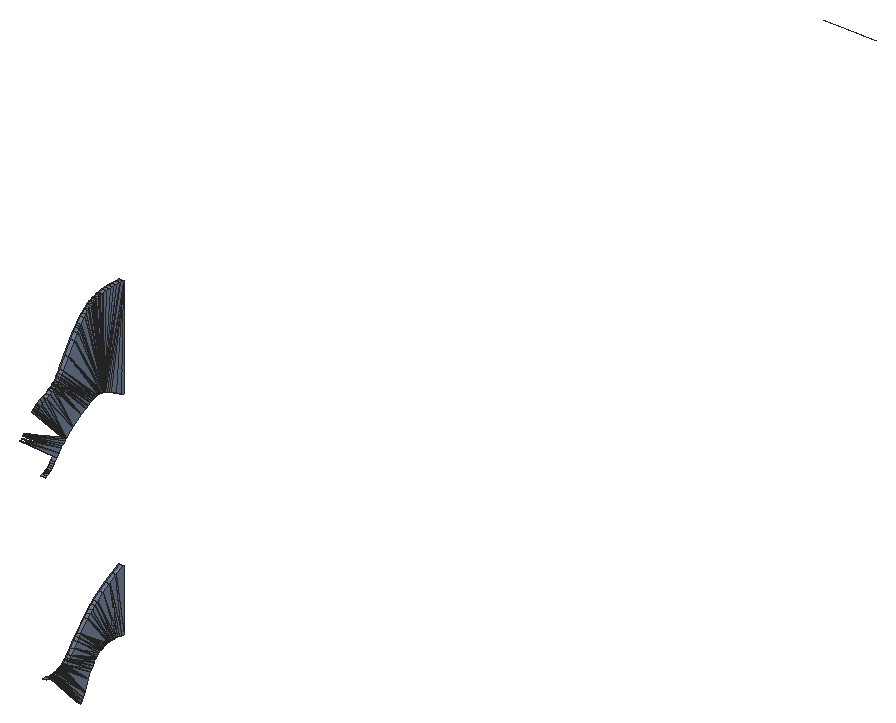
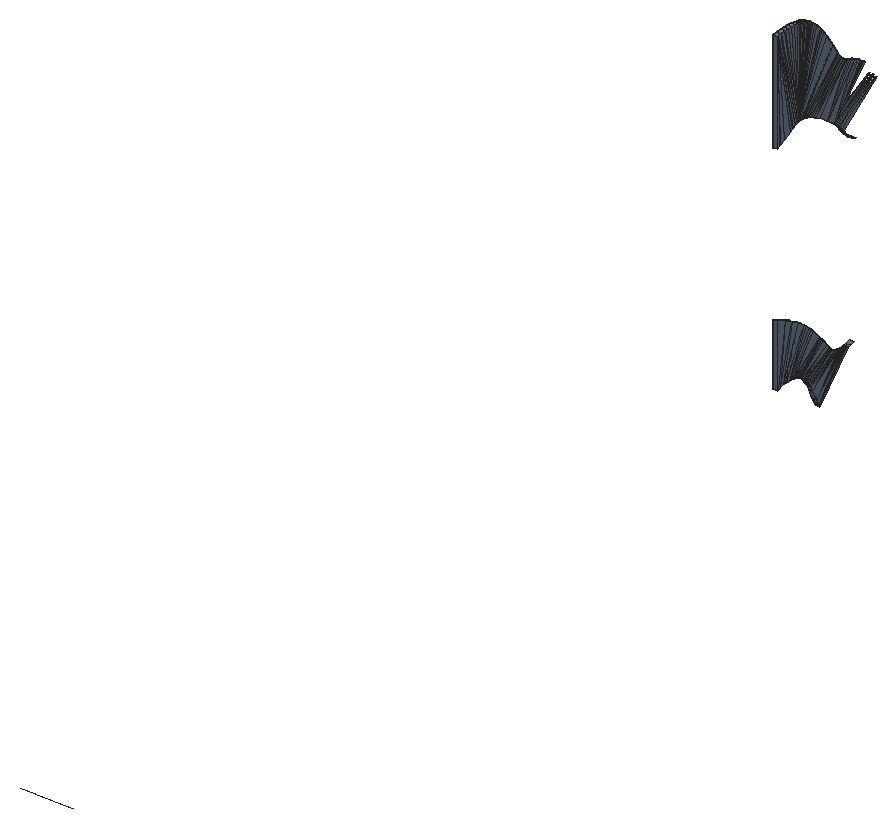
# SketchUp Ruby script. Lengths in inches.
U = 1.inch
M = Sketchup.active_model
def pt(a) = Geom::Point3d.new(a.map { |v| v * U })
def face(e, loops, mat)
  f = e.add_face(loops[0].map { |a| pt(a) })
  loops[1..].each { |l| e.add_face(l.map { |a| pt(a) }).erase! }
  f.material = f.back_material = mat if mat
  f
end
# faces: each face lists its corners as indices into pts; further lists are holes
def faces(e, pts, list, mat = nil) = list.each { |f| face(e, (f[0].is_a?(Array) ? f : [f]).map { |l| l.map { |i| pts[i] } }, mat) }
# xy, xz, yz: faces in a plane at the given z, y or x. An outline is a flat list of corners, or four numbers for a rectangle; further outlines are holes
def ring(l) = l.size == 4 ? [[l[0], l[1]], [l[2], l[1]], [l[2], l[3]], [l[0], l[3]]] : l.each_slice(2).to_a
def flat(e, list, mat, &to3) = list.each { |f| face(e, (f[0].is_a?(Array) ? f : [f]).map { |l| ring(l).map { |u, v| to3.(u, v) } }, mat) }
def xy(e, z, list, mat = nil) = flat(e, list, mat) { |x, y| [x, y, z] }
def xz(e, y, list, mat = nil) = flat(e, list, mat) { |x, z| [x, y, z] }
def yz(e, x, list, mat = nil) = flat(e, list, mat) { |y, z| [x, y, z] }
def lines(e, pts, list) = list.each { |a, b| e.add_line(pt(pts[a]), pt(pts[b])) }
# prism: a flat outline (further loops are holes) pulled along v
def prism(e, loops, v, mat = nil)
  f = face(e, loops, mat); d = Geom::Vector3d.new(v.map { |x| x * U })
  f.pushpull(f.normal.samedirection?(d) ? d.length : -d.length)
end
def box(e, o, s, mat = nil) = prism(e, [[o, [o[0] + s[0], o[1], o[2]], [o[0] + s[0], o[1] + s[1], o[2]], [o[0], o[1] + s[1], o[2]]]], [0, 0, s[2]], mat)
def at(x, y, z, deg = 0) = Geom::Transformation.translation(pt([x, y, z])) * Geom::Transformation.rotation(ORIGIN, Z_AXIS, deg.degrees)
def axes(o, x, y, z) = Geom::Transformation.new([*x, 0, *y, 0, *z, 0, *pt(o).to_a, 1])
def part(name) = M.definitions.add(name)
# library, detail: a bought-in or finely detailed component or shape, given as its bounding box
def library(name, o, s) = part(name).tap { |d| box(d.entities, o, s) }
def detail(e, o, s) = box(e.add_group.entities, o, s)
def put(e, d, t, mat = nil) = e.add_instance(d, t).tap { |i| i.material = mat if mat }
def group(e, t, mat = nil) = e.add_group.tap { |g| g.transformation = t; g.material = mat if mat }.entities
root = M.entities
M.materials.add("3D66_SU_1584934530605_002").color = [112, 126, 151]
xy(root,51.61,[[122.5,316.66,123.07,316.78],[122.5,316.78,123.07,316.85],[122.5,316.85,123.07,316.91]],"3D66_SU_1584934530605_002")
xy(root,51.62,[[122.5,316.97,123.07,317.03]],"3D66_SU_1584934530605_002")
xy(root,80.71,[[122.5,323.52,123.07,323.66],[122.5,323.66,123.07,323.8]],"3D66_SU_1584934530605_002")
xz(root,327.5625,[[122.5,51.65,123.07,59.52],[122.5,79.03,123.07,91.85]],"3D66_SU_1584934530605_002")
yz(root,122.5,[[320.78,46.84,316.4,51.64,316.53,51.625],[320.78,46.84,316.53,51.625,316.66,51.61],[320.78,46.84,316.66,51.61,316.78,51.61],[320.78,46.84,316.78,51.61,316.85,51.61],[320.78,46.84,316.85,51.61,316.91,51.61],
  [320.78,46.84,316.91,51.61,320.92,47.07],[320.92,47.07,316.91,51.61,316.97,51.62],[320.92,47.07,316.97,51.62,321.05,47.33],[321.05,47.33,316.97,51.62,317.03,51.62],[321.05,47.33,317.03,51.62,321.34,47.89],
  [321.34,47.89,317.03,51.62,317.28,51.66],[321.34,47.89,317.28,51.66,317.4,51.68],[321.34,47.89,317.4,51.68,317.51,51.71],[321.34,47.89,317.51,51.71,317.63,51.74],[321.34,47.89,317.63,51.74,317.74,51.78],
  [321.34,47.89,317.74,51.78,317.85,51.82],[321.34,47.89,317.85,51.82,317.96,51.86],[321.34,47.89,317.96,51.86,318.07,51.91],[321.34,47.89,318.07,51.91,321.94,49.14],[321.94,49.14,318.07,51.91,318.18,51.97],
  [321.94,49.14,318.18,51.97,318.29,52.03],[321.94,49.14,318.29,52.03,318.4,52.09],[321.94,49.14,318.4,52.09,318.51,52.16],[321.94,49.14,318.51,52.16,322.27,49.75],[322.27,49.75,318.51,52.16,318.625,52.24],
  [322.27,49.75,318.625,52.24,322.4375,50.04],[322.4375,50.04,318.625,52.24,318.86,52.42],[322.4375,50.04,318.86,52.42,318.97,52.52],[322.4375,50.04,318.97,52.52,322.62,50.32],[322.62,50.32,318.97,52.52,319.09,52.64],
  [322.62,50.32,319.09,52.64,322.8,50.57],[322.8,50.57,319.09,52.64,322.9,50.6875],[322.9,50.6875,319.09,52.64,319.3125,52.88],[322.9,50.6875,319.3125,52.88,322.99,50.8],[322.99,50.8,319.3125,52.88,323.09,50.9],
  [323.09,50.9,319.3125,52.88,323.19,51],[323.19,51,319.3125,52.88,323.3,51.09],[323.3,51.09,319.3125,52.88,319.77,53.46],[323.3,51.09,319.77,53.46,323.4,51.17],[323.4,51.17,319.77,53.46,323.62,51.3125],
  [323.62,51.3125,319.77,53.46,320.25,54.08],[323.62,51.3125,320.25,54.08,323.84,51.4375],[323.84,51.4375,320.25,54.08,320.5,54.4],[323.84,51.4375,320.5,54.4,323.95,51.5],[323.95,51.5,320.5,54.4,324.0625,51.55],
  [324.0625,51.55,320.5,54.4,320.78,54.71],[324.0625,51.55,320.78,54.71,324.18,51.6],[324.18,51.6,320.78,54.71,324.3,51.65],[324.3,51.65,320.78,54.71,324.42,51.69],[327.5625,51.65,326.38,58.99,327.5625,59.52],
  [327.5625,51.65,327.26,51.73,326.38,58.99],[324.42,51.69,320.78,54.71,324.54,51.73],[324.54,51.73,320.78,54.71,324.66,51.77],[327.26,51.73,325.29,58.43,326.38,58.99],[327.26,51.73,326.96,51.8,325.29,58.43],
  [324.66,51.77,320.78,54.71,324.78,51.8],[324.78,51.8,320.78,54.71,324.91,51.83],[326.96,51.8,326.67,51.85,325.29,58.43],[324.91,51.83,320.78,54.71,325.03,51.85],[325.03,51.85,320.78,54.71,321.95,55.99],
  [325.03,51.85,321.95,55.99,325.16,51.875],[326.67,51.85,324.3,57.86,325.29,58.43],[326.67,51.85,326.38,51.89,324.3,57.86],[325.16,51.875,321.95,55.99,325.29,51.89],[325.29,51.89,321.95,55.99,322.28,56.32],
  [325.29,51.89,322.28,56.32,325.42,51.9],[326.38,51.89,323.4,57.27,324.3,57.86],[326.38,51.89,326.1,51.91,323.4,57.27],[325.42,51.9,322.28,56.32,322.625,56.64],[325.42,51.9,322.625,56.64,325.55,51.91],
  [325.55,51.91,322.625,56.64,323,56.96],[325.55,51.91,323,56.96,325.82,51.92],[326.1,51.91,325.82,51.92,323.4,57.27],[325.82,51.92,323,56.96,323.4,57.27],[316.98,76.43,311.9,80.33,317.3,76.82],
  [317.3,76.82,312.09,80.52,317.64,77.21],[317.64,77.21,312.27,80.74,317.82,77.41],[317.82,77.41,312.38,80.9,318.02,77.59],[318.02,77.59,312.38,80.9,318.24,77.78],[318.24,77.78,312.38,80.9,318.47,77.96],
  [318.47,77.96,313.73,82.9,313.8125,82.97],[318.47,77.96,313.8125,82.97,313.89,83.03],[318.47,77.96,313.89,83.03,313.98,83.1],[318.47,77.96,313.98,83.1,314.16,83.22],[318.47,77.96,314.16,83.22,314.36,83.33],
  [318.47,77.96,314.36,83.33,314.56,83.4375],[318.47,77.96,314.56,83.4375,314.99,83.64],[318.47,77.96,314.99,83.64,315.43,83.82],[318.47,77.96,315.43,83.82,319.57,78.75],[319.57,78.75,315.43,83.82,315.87,84.01],
  [319.57,78.75,315.87,84.01,316.3,84.2],[319.57,78.75,316.3,84.2,316.5,84.31],[319.57,78.75,316.5,84.31,320.84,79.61],[327.5625,79.03,327.3,79.14,327.5625,91.85],[327.3,79.14,327.05,79.27,327.5625,91.85],
  [327.05,79.27,326.54,79.55,327.5625,91.85],[326.54,79.55,325.52,80.14,327.5625,91.85],[320.84,79.61,316.5,84.31,316.6875,84.41],[320.84,79.61,316.6875,84.41,316.87,84.53],[320.84,79.61,316.87,84.53,316.95,84.59],
  [320.84,79.61,316.95,84.59,321.5,79.99],[321.5,79.99,316.95,84.59,317.03,84.65],[321.5,79.99,317.03,84.65,317.1875,84.78],[321.5,79.99,317.1875,84.78,321.83,80.17],[325.52,80.14,325.26,80.27,327.5625,91.85],
  [321.83,80.17,317.1875,84.78,317.33,84.92],[321.83,80.17,317.33,84.92,322.16,80.32],[325.26,80.27,325,80.39,327.5625,91.85],[322.16,80.32,317.33,84.92,317.46,85.06],[322.16,80.32,317.46,85.06,317.59,85.2],
  [322.16,80.32,317.59,85.2,322.48,80.45],[325,80.39,324.74,80.5,327.5625,91.85],[322.48,80.45,317.59,85.2,322.63,80.51],[324.74,80.5,324.61,80.55,327.5625,91.85],[322.63,80.51,317.59,85.2,317.82,85.49],
  [322.63,80.51,317.82,85.49,322.79,80.5625],[324.61,80.55,324.48,80.59,327.5625,91.85],[322.79,80.5625,317.82,85.49,322.94,80.61],[324.48,80.59,324.35,80.625,326.96,91.92],[324.48,80.59,326.96,91.92,327.5625,91.85],
  [322.94,80.61,317.82,85.49,318.03,85.79],[322.94,80.61,318.03,85.79,323.09,80.64],[324.35,80.625,324.21,80.65,326.38,91.96],[324.35,80.625,326.38,91.96,326.96,91.92],[323.09,80.64,318.03,85.79,323.24,80.67],
  [324.21,80.65,319.77,88.49,320.25,89.21],[324.21,80.65,324.08,80.68,319.77,88.49],[324.21,80.65,320.25,89.21,320.5,89.54],[324.21,80.65,320.5,89.54,320.64,89.7],[324.21,80.65,320.64,89.7,320.78,89.84],
  [324.21,80.65,320.78,89.84,321.35,90.4],[324.21,80.65,321.35,90.4,321.64,90.67],[324.21,80.65,321.64,90.67,321.95,90.92],[324.21,80.65,321.95,90.92,322.11,91.03],[324.21,80.65,322.11,91.03,322.28,91.14],
  [324.21,80.65,322.28,91.14,322.45,91.25],[324.21,80.65,322.45,91.25,322.625,91.35],[324.21,80.65,322.625,91.35,322.81,91.4375],[324.21,80.65,322.81,91.4375,323,91.52],[324.21,80.65,323,91.52,323.2,91.6],
  [324.21,80.65,323.2,91.6,323.4,91.66],[324.21,80.65,323.4,91.66,323.62,91.72],[324.21,80.65,323.62,91.72,323.84,91.78],[324.21,80.65,323.84,91.78,324.07,91.82],[324.21,80.65,324.07,91.82,324.3,91.86],
  [324.21,80.65,324.3,91.86,324.78,91.93],[324.21,80.65,324.78,91.93,325.29,91.96],[324.21,80.65,325.29,91.96,325.82,91.97],[324.21,80.65,325.82,91.97,326.38,91.96],[323.24,80.67,318.03,85.79,323.38,80.69],
  [324.08,80.68,318.86,87.07,319.77,88.49],[324.08,80.68,323.94,80.7,318.86,87.07],[323.38,80.69,318.03,85.79,323.52,80.71],[323.94,80.7,323.8,80.71,318.86,87.07],[323.52,80.71,318.03,85.79,318.86,87.07],
  [323.52,80.71,318.86,87.07,323.66,80.71],[323.66,80.71,318.86,87.07,323.8,80.71]],"3D66_SU_1584934530605_002")
yz(root,123.07,[[320.78,46.84,316.53,51.625,316.4,51.64],[320.78,46.84,316.66,51.61,316.53,51.625],[320.78,46.84,316.78,51.61,316.66,51.61],[320.78,46.84,316.85,51.61,316.78,51.61],[320.78,46.84,316.91,51.61,316.85,51.61],
  [320.78,46.84,320.92,47.07,316.91,51.61],[320.92,47.07,316.97,51.62,316.91,51.61],[320.92,47.07,321.05,47.33,316.97,51.62],[321.05,47.33,317.03,51.62,316.97,51.62],[321.05,47.33,321.34,47.89,317.03,51.62],
  [321.34,47.89,317.28,51.66,317.03,51.62],[321.34,47.89,317.4,51.68,317.28,51.66],[321.34,47.89,317.51,51.71,317.4,51.68],[321.34,47.89,317.63,51.74,317.51,51.71],[321.34,47.89,317.74,51.78,317.63,51.74],
  [321.34,47.89,317.85,51.82,317.74,51.78],[321.34,47.89,317.96,51.86,317.85,51.82],[321.34,47.89,318.07,51.91,317.96,51.86],[321.34,47.89,321.94,49.14,318.07,51.91],[321.94,49.14,318.18,51.97,318.07,51.91],
  [321.94,49.14,318.29,52.03,318.18,51.97],[321.94,49.14,318.4,52.09,318.29,52.03],[321.94,49.14,318.51,52.16,318.4,52.09],[321.94,49.14,322.27,49.75,318.51,52.16],[322.27,49.75,318.625,52.24,318.51,52.16],
  [322.27,49.75,322.4375,50.04,318.625,52.24],[322.4375,50.04,318.86,52.42,318.625,52.24],[322.4375,50.04,318.97,52.52,318.86,52.42],[322.4375,50.04,322.62,50.32,318.97,52.52],[322.62,50.32,319.09,52.64,318.97,52.52],
  [322.62,50.32,322.8,50.57,319.09,52.64],[322.8,50.57,322.9,50.6875,319.09,52.64],[322.9,50.6875,319.3125,52.88,319.09,52.64],[322.9,50.6875,322.99,50.8,319.3125,52.88],[322.99,50.8,323.09,50.9,319.3125,52.88],
  [323.09,50.9,323.19,51,319.3125,52.88],[323.19,51,323.3,51.09,319.3125,52.88],[323.3,51.09,319.77,53.46,319.3125,52.88],[323.3,51.09,323.4,51.17,319.77,53.46],[323.4,51.17,323.62,51.3125,319.77,53.46],
  [323.62,51.3125,320.25,54.08,319.77,53.46],[323.62,51.3125,323.84,51.4375,320.25,54.08],[323.84,51.4375,320.5,54.4,320.25,54.08],[323.84,51.4375,323.95,51.5,320.5,54.4],[323.95,51.5,324.0625,51.55,320.5,54.4],
  [324.0625,51.55,320.78,54.71,320.5,54.4],[324.0625,51.55,324.18,51.6,320.78,54.71],[324.18,51.6,324.3,51.65,320.78,54.71],[324.3,51.65,324.42,51.69,320.78,54.71],[327.5625,51.65,326.38,58.99,327.26,51.73],
  [327.5625,51.65,327.5625,59.52,326.38,58.99],[324.42,51.69,324.54,51.73,320.78,54.71],[324.54,51.73,324.66,51.77,320.78,54.71],[327.26,51.73,325.29,58.43,326.96,51.8],[327.26,51.73,326.38,58.99,325.29,58.43],
  [324.66,51.77,324.78,51.8,320.78,54.71],[324.78,51.8,324.91,51.83,320.78,54.71],[326.96,51.8,325.29,58.43,326.67,51.85],[324.91,51.83,325.03,51.85,320.78,54.71],[325.03,51.85,321.95,55.99,320.78,54.71],
  [325.03,51.85,325.16,51.875,321.95,55.99],[326.67,51.85,324.3,57.86,326.38,51.89],[326.67,51.85,325.29,58.43,324.3,57.86],[325.16,51.875,325.29,51.89,321.95,55.99],[325.29,51.89,322.28,56.32,321.95,55.99],
  [325.29,51.89,325.42,51.9,322.28,56.32],[326.38,51.89,323.4,57.27,326.1,51.91],[326.38,51.89,324.3,57.86,323.4,57.27],[325.42,51.9,322.625,56.64,322.28,56.32],[325.42,51.9,325.55,51.91,322.625,56.64],
  [325.55,51.91,323,56.96,322.625,56.64],[325.55,51.91,325.82,51.92,323,56.96],[326.1,51.91,323.4,57.27,325.82,51.92],[325.82,51.92,323.4,57.27,323,56.96],[316.98,76.43,317.3,76.82,311.9,80.33],
  [317.3,76.82,317.64,77.21,312.09,80.52],[317.64,77.21,317.82,77.41,312.27,80.74],[317.82,77.41,318.02,77.59,312.38,80.9],[318.02,77.59,318.24,77.78,312.38,80.9],[318.24,77.78,318.47,77.96,312.38,80.9],
  [318.47,77.96,313.8125,82.97,313.73,82.9],[318.47,77.96,313.89,83.03,313.8125,82.97],[318.47,77.96,313.98,83.1,313.89,83.03],[318.47,77.96,314.16,83.22,313.98,83.1],[318.47,77.96,314.36,83.33,314.16,83.22],
  [318.47,77.96,314.56,83.4375,314.36,83.33],[318.47,77.96,314.99,83.64,314.56,83.4375],[318.47,77.96,315.43,83.82,314.99,83.64],[318.47,77.96,319.57,78.75,315.43,83.82],[319.57,78.75,315.87,84.01,315.43,83.82],
  [319.57,78.75,316.3,84.2,315.87,84.01],[319.57,78.75,316.5,84.31,316.3,84.2],[319.57,78.75,320.84,79.61,316.5,84.31],[327.5625,79.03,327.5625,91.85,327.3,79.14],[327.3,79.14,327.5625,91.85,327.05,79.27],
  [327.05,79.27,327.5625,91.85,326.54,79.55],[326.54,79.55,327.5625,91.85,325.52,80.14],[320.84,79.61,316.6875,84.41,316.5,84.31],[320.84,79.61,316.87,84.53,316.6875,84.41],[320.84,79.61,316.95,84.59,316.87,84.53],
  [320.84,79.61,321.5,79.99,316.95,84.59],[321.5,79.99,317.03,84.65,316.95,84.59],[321.5,79.99,317.1875,84.78,317.03,84.65],[321.5,79.99,321.83,80.17,317.1875,84.78],[325.52,80.14,327.5625,91.85,325.26,80.27],
  [321.83,80.17,317.33,84.92,317.1875,84.78],[321.83,80.17,322.16,80.32,317.33,84.92],[325.26,80.27,327.5625,91.85,325,80.39],[322.16,80.32,317.46,85.06,317.33,84.92],[322.16,80.32,317.59,85.2,317.46,85.06],
  [322.16,80.32,322.48,80.45,317.59,85.2],[325,80.39,327.5625,91.85,324.74,80.5],[322.48,80.45,322.63,80.51,317.59,85.2],[324.74,80.5,327.5625,91.85,324.61,80.55],[322.63,80.51,317.82,85.49,317.59,85.2],
  [322.63,80.51,322.79,80.5625,317.82,85.49],[324.61,80.55,327.5625,91.85,324.48,80.59],[322.79,80.5625,322.94,80.61,317.82,85.49],[324.48,80.59,326.96,91.92,324.35,80.625],[324.48,80.59,327.5625,91.85,326.96,91.92],
  [322.94,80.61,318.03,85.79,317.82,85.49],[322.94,80.61,323.09,80.64,318.03,85.79],[324.35,80.625,326.38,91.96,324.21,80.65],[324.35,80.625,326.96,91.92,326.38,91.96],[323.09,80.64,323.24,80.67,318.03,85.79],
  [324.21,80.65,319.77,88.49,324.08,80.68],[324.21,80.65,320.25,89.21,319.77,88.49],[324.21,80.65,320.5,89.54,320.25,89.21],[324.21,80.65,320.64,89.7,320.5,89.54],[324.21,80.65,320.78,89.84,320.64,89.7],
  [324.21,80.65,321.35,90.4,320.78,89.84],[324.21,80.65,321.64,90.67,321.35,90.4],[324.21,80.65,321.95,90.92,321.64,90.67],[324.21,80.65,322.11,91.03,321.95,90.92],[324.21,80.65,322.28,91.14,322.11,91.03],
  [324.21,80.65,322.45,91.25,322.28,91.14],[324.21,80.65,322.625,91.35,322.45,91.25],[324.21,80.65,322.81,91.4375,322.625,91.35],[324.21,80.65,323,91.52,322.81,91.4375],[324.21,80.65,323.2,91.6,323,91.52],
  [324.21,80.65,323.4,91.66,323.2,91.6],[324.21,80.65,323.62,91.72,323.4,91.66],[324.21,80.65,323.84,91.78,323.62,91.72],[324.21,80.65,324.07,91.82,323.84,91.78],[324.21,80.65,324.3,91.86,324.07,91.82],
  [324.21,80.65,324.78,91.93,324.3,91.86],[324.21,80.65,325.29,91.96,324.78,91.93],[324.21,80.65,325.82,91.97,325.29,91.96],[324.21,80.65,326.38,91.96,325.82,91.97],[323.24,80.67,323.38,80.69,318.03,85.79],
  [324.08,80.68,318.86,87.07,323.94,80.7],[324.08,80.68,319.77,88.49,318.86,87.07],[323.38,80.69,323.52,80.71,318.03,85.79],[323.94,80.7,318.86,87.07,323.8,80.71],[323.52,80.71,318.86,87.07,318.03,85.79],
  [323.52,80.71,323.66,80.71,318.86,87.07],[323.66,80.71,323.8,80.71,318.86,87.07]],"3D66_SU_1584934530605_002")
p = [[123.07,320.78,46.84],[122.5,320.78,46.84],[122.5,320.92,47.07],[123.07,320.92,47.07],[122.5,321.05,47.33],[123.07,321.05,47.33],
  [122.5,321.34,47.89],[123.07,321.34,47.89],[122.5,321.94,49.14],[123.07,321.94,49.14],[122.5,322.27,49.75],[123.07,322.27,49.75],
  [122.5,322.4375,50.04],[123.07,322.4375,50.04],[122.5,322.62,50.32],[123.07,322.62,50.32],[122.5,322.8,50.57],[123.07,322.8,50.57],
  [122.5,322.9,50.6875],[123.07,322.9,50.6875],[122.5,322.99,50.8],[123.07,322.99,50.8],[122.5,323.09,50.9],[123.07,323.09,50.9],
  [122.5,323.19,51],[123.07,323.19,51],[122.5,323.3,51.09],[123.07,323.3,51.09],[122.5,323.4,51.17],[123.07,323.4,51.17],
  [122.5,323.62,51.3125],[123.07,323.62,51.3125],[122.5,323.84,51.4375],[123.07,323.84,51.4375],[122.5,323.95,51.5],[123.07,323.95,51.5],
  [122.5,324.0625,51.55],[123.07,324.0625,51.55],[123.07,316.4,51.64],[122.5,316.4,51.64],[122.5,316.27,51.67],[123.07,316.27,51.67],
  [123.07,316.53,51.625],[122.5,316.53,51.625],[123.07,316.66,51.61],[122.5,316.66,51.61],[123.07,316.97,51.62],[122.5,316.97,51.62],
  [122.5,316.91,51.61],[123.07,316.91,51.61],[123.07,317.28,51.66],[122.5,317.28,51.66],[122.5,317.03,51.62],[123.07,317.03,51.62],
  [122.5,324.18,51.6],[123.07,324.18,51.6],[122.5,324.3,51.65],[123.07,324.3,51.65],[122.5,324.42,51.69],[123.07,324.42,51.69],
  [123.07,327.26,51.73],[122.5,327.26,51.73],[122.5,327.5625,51.65],[123.07,327.5625,51.65],[123.07,316.01,51.72],[122.5,316.01,51.72],
  [122.5,315.45,51.84],[123.07,315.45,51.84],[123.07,317.4,51.68],[122.5,317.4,51.68],[123.07,317.51,51.71],[122.5,317.51,51.71],
  [123.07,317.63,51.74],[122.5,317.63,51.74],[123.07,317.74,51.78],[122.5,317.74,51.78],[122.5,324.54,51.73],[123.07,324.54,51.73],
  [122.5,324.66,51.77],[123.07,324.66,51.77],[123.07,326.96,51.8],[122.5,326.96,51.8],[123.07,317.85,51.82],[122.5,317.85,51.82],
  [123.07,317.96,51.86],[122.5,317.96,51.86],[122.5,324.78,51.8],[123.07,324.78,51.8],[122.5,324.91,51.83],[123.07,324.91,51.83],
  [122.5,325.03,51.85],[123.07,325.03,51.85],[123.07,326.67,51.85],[122.5,326.67,51.85],[123.07,318.07,51.91],[122.5,318.07,51.91],
  [123.07,318.18,51.97],[122.5,318.18,51.97],[122.5,325.16,51.875],[123.07,325.16,51.875],[122.5,325.29,51.89],[123.07,325.29,51.89],
  [122.5,325.42,51.9],[123.07,325.42,51.9],[122.5,325.55,51.91],[123.07,325.55,51.91],[122.5,325.82,51.92],[123.07,325.82,51.92],
  [122.5,326.1,51.91],[123.07,326.1,51.91],[122.5,326.38,51.89],[123.07,326.38,51.89],[123.07,318.29,52.03],[122.5,318.29,52.03],
  [122.5,318.4,52.09],[123.07,318.4,52.09],[123.07,318.51,52.16],[122.5,318.51,52.16],[123.07,318.625,52.24],[122.5,318.625,52.24],
  [123.07,318.86,52.42],[122.5,318.86,52.42],[123.07,318.97,52.52],[122.5,318.97,52.52],[123.07,319.09,52.64],[122.5,319.09,52.64],
  [123.07,319.3125,52.88],[122.5,319.3125,52.88],[123.07,319.77,53.46],[122.5,319.77,53.46],[123.07,320.25,54.08],[122.5,320.25,54.08],
  [123.07,320.5,54.4],[122.5,320.5,54.4],[123.07,320.78,54.71],[122.5,320.78,54.71],[123.07,321.95,55.99],[122.5,321.95,55.99],
  [123.07,322.28,56.32],[122.5,322.28,56.32],[123.07,322.625,56.64],[122.5,322.625,56.64],[123.07,323,56.96],[122.5,323,56.96],
  [123.07,323.4,57.27],[122.5,323.4,57.27],[123.07,324.3,57.86],[122.5,324.3,57.86],[123.07,325.29,58.43],[122.5,325.29,58.43],
  [123.07,326.38,58.99],[122.5,326.38,58.99],[123.07,327.5625,59.52],[122.5,327.5625,59.52],[123.07,315.22,74.94],[122.5,315.22,74.94],
  [122.5,315.43,75.03],[123.07,315.43,75.03],[122.5,315.64,75.14],[123.07,315.64,75.14],[123.07,315.74,75.2],[122.5,315.74,75.2],
  [123.07,315.84,75.26],[122.5,315.84,75.26],[122.5,315.93,75.33],[123.07,315.93,75.33],[123.07,316.02,75.4],[122.5,316.02,75.4],
  [122.5,316.2,75.55],[123.07,316.2,75.55],[122.5,316.36,75.71],[123.07,316.36,75.71],[122.5,316.52,75.88],[123.07,316.52,75.88],
  [122.5,316.68,76.06],[123.07,316.68,76.06],[122.5,316.98,76.43],[123.07,316.98,76.43],[122.5,317.3,76.82],[123.07,317.3,76.82],
  [122.5,317.64,77.21],[123.07,317.64,77.21],[122.5,317.82,77.41],[123.07,317.82,77.41],[122.5,318.02,77.59],[123.07,318.02,77.59],
  [122.5,318.24,77.78],[123.07,318.24,77.78],[122.5,318.47,77.96],[123.07,318.47,77.96],[122.5,319.57,78.75],[123.07,319.57,78.75],
  [122.5,320.84,79.61],[123.07,320.84,79.61],[123.07,327.3,79.14],[122.5,327.3,79.14],[122.5,327.5625,79.03],[123.07,327.5625,79.03],
  [123.07,327.05,79.27],[122.5,327.05,79.27],[123.07,326.54,79.55],[122.5,326.54,79.55],[123.07,325.52,80.14],[122.5,325.52,80.14],
  [122.5,321.5,79.99],[123.07,321.5,79.99],[122.5,321.83,80.17],[123.07,321.83,80.17],[123.07,325.26,80.27],[122.5,325.26,80.27],
  [122.5,322.16,80.32],[123.07,322.16,80.32],[122.5,322.48,80.45],[123.07,322.48,80.45],[123.07,325,80.39],[122.5,325,80.39],
  [123.07,324.74,80.5],[122.5,324.74,80.5],[122.5,322.63,80.51],[123.07,322.63,80.51],[122.5,322.79,80.5625],[123.07,322.79,80.5625],
  [123.07,324.48,80.59],[122.5,324.48,80.59],[122.5,324.61,80.55],[123.07,324.61,80.55],[122.5,322.94,80.61],[123.07,322.94,80.61],
  [122.5,323.09,80.64],[123.07,323.09,80.64],[122.5,323.24,80.67],[123.07,323.24,80.67],[123.07,324.21,80.65],[122.5,324.21,80.65],
  [122.5,324.35,80.625],[123.07,324.35,80.625],[122.5,323.38,80.69],[123.07,323.38,80.69],[122.5,323.52,80.71],[123.07,323.52,80.71],
  [123.07,323.8,80.71],[122.5,323.8,80.71],[122.5,323.94,80.7],[123.07,323.94,80.7],[122.5,324.08,80.68],[123.07,324.08,80.68],
  [123.07,315.87,84.01],[122.5,315.87,84.01],[122.5,315.43,83.82],[123.07,315.43,83.82],[123.07,316.3,84.2],[122.5,316.3,84.2],
  [123.07,316.5,84.31],[122.5,316.5,84.31],[123.07,316.6875,84.41],[122.5,316.6875,84.41],[123.07,316.87,84.53],[122.5,316.87,84.53],
  [122.5,316.95,84.59],[123.07,316.95,84.59],[122.5,317.03,84.65],[123.07,317.03,84.65],[123.07,317.1875,84.78],[122.5,317.1875,84.78],
  [123.07,317.33,84.92],[122.5,317.33,84.92],[123.07,317.46,85.06],[122.5,317.46,85.06],[123.07,317.59,85.2],[122.5,317.59,85.2],
  [123.07,317.82,85.49],[122.5,317.82,85.49],[123.07,318.03,85.79],[122.5,318.03,85.79],[123.07,318.86,87.07],[122.5,318.86,87.07],
  [123.07,319.77,88.49],[122.5,319.77,88.49],[123.07,320.25,89.21],[122.5,320.25,89.21],[123.07,320.5,89.54],[122.5,320.5,89.54],
  [123.07,320.64,89.7],[122.5,320.64,89.7],[123.07,320.78,89.84],[122.5,320.78,89.84],[123.07,321.35,90.4],[122.5,321.35,90.4],
  [123.07,321.64,90.67],[122.5,321.64,90.67],[123.07,321.95,90.92],[122.5,321.95,90.92],[123.07,322.11,91.03],[122.5,322.11,91.03],
  [123.07,322.28,91.14],[122.5,322.28,91.14],[123.07,322.45,91.25],[122.5,322.45,91.25],[123.07,322.625,91.35],[122.5,322.625,91.35],
  [123.07,322.81,91.4375],[122.5,322.81,91.4375],[123.07,323,91.52],[122.5,323,91.52],[123.07,323.2,91.6],[122.5,323.2,91.6],
  [123.07,323.4,91.66],[122.5,323.4,91.66],[123.07,323.62,91.72],[122.5,323.62,91.72],[123.07,323.84,91.78],[122.5,323.84,91.78],
  [123.07,324.07,91.82],[122.5,324.07,91.82],[123.07,324.3,91.86],[122.5,324.3,91.86],[123.07,327.5625,91.85],[122.5,327.5625,91.85],
  [122.5,326.96,91.92],[123.07,326.96,91.92],[123.07,324.78,91.93],[122.5,324.78,91.93],[123.07,325.29,91.96],[122.5,325.29,91.96],
  [122.5,326.38,91.96],[123.07,326.38,91.96],[123.07,325.82,91.97],[122.5,325.82,91.97],[111.875,452.39,62.71],[118.5625,452.39,62.71]]
faces(root,p,[[0,1,2,3],[3,2,4,5],[5,4,6,7],[7,6,8,9],[9,8,10,11],[11,10,12,13],[13,12,14,15],[15,14,16,17],
  [17,16,18,19],[19,18,20,21],[21,20,22,23],[23,22,24,25],[25,24,26,27],[27,26,28,29],[29,28,30,31],[31,30,32,33],
  [33,32,34,35],[35,34,36,37],[38,39,40,41],[42,43,39,38],[44,45,43,42],[46,47,48,49],[50,51,52,53],[37,36,54,55],
  [55,54,56,57],[57,56,58,59],[60,61,62,63],[64,65,66,67],[41,40,65,64],[68,69,51,50],[70,71,69,68],[72,73,71,70],
  [74,75,73,72],[59,58,76,77],[77,76,78,79],[80,81,61,60],[82,83,75,74],[84,85,83,82],[79,78,86,87],[87,86,88,89],
  [89,88,90,91],[92,93,81,80],[94,95,85,84],[96,97,95,94],[91,90,98,99],[99,98,100,101],[101,100,102,103],[103,102,104,105],
  [105,104,106,107],[107,106,108,109],[109,108,110,111],[111,110,93,92],[112,113,97,96],[114,113,112],[114,112,115],[116,117,114,115],
  [118,119,117,116],[120,121,119,118],[122,123,121,120],[124,125,123,122],[126,127,125,124],[128,129,127,126],[130,131,129,128],[132,133,131,130],
  [134,135,133,132],[136,137,135,134],[138,139,137,136],[140,141,139,138],[142,143,141,140],[144,145,143,142],[146,147,145,144],[148,149,147,146],
  [150,151,149,148],[152,153,151,150],[154,155,156,157],[157,156,158,159],[158,160,159],[158,161,160],[161,162,160],[161,163,162],
  [162,163,164,165],[164,166,165],[164,167,166],[166,167,168,169],[169,168,170,171],[171,170,172,173],[173,172,174,175],[175,174,176,177],
  [177,176,178,179],[179,178,180,181],[181,180,182,183],[183,182,184,185],[185,184,186,187],[187,186,188,189],[189,188,190,191],[191,190,192,193],
  [194,195,196,197],[198,199,195,194],[200,201,199,198],[202,203,201,200],[193,192,204,205],[205,204,206,207],[208,209,203,202],[207,206,210,211],
  [211,210,212,213],[214,215,209,208],[216,217,215,214],[213,212,218,219],[219,218,220,221],[222,223,224,225],[225,224,217,216],[221,220,226,227],
  [227,226,228,229],[229,228,230,231],[232,233,234,235],[235,234,223,222],[231,230,236,237],[237,236,238,239],[240,241,242,243],[243,242,244,245],
  [245,244,233,232],[246,247,248,249],[250,251,247,246],[252,253,251,250],[254,255,253,252],[256,257,255,254],[258,257,256],[258,256,259],
  [260,258,259],[260,259,261],[262,263,260,261],[264,265,263,262],[266,267,265,264],[268,269,267,266],[270,271,269,268],[272,273,271,270],
  [274,275,273,272],[276,277,275,274],[278,279,277,276],[280,281,279,278],[282,283,281,280],[284,285,283,282],[286,287,285,284],[288,289,287,286],
  [290,291,289,288],[292,293,291,290],[294,295,293,292],[296,297,295,294],[298,299,297,296],[300,301,299,298],[302,303,301,300],[304,305,303,302],
  [306,307,305,304],[308,309,307,306],[310,311,309,308],[312,313,311,310],[314,315,313,312],[316,317,318,319],[320,321,315,314],[322,323,321,320],
  [319,318,324,325],[326,327,323,322],[325,324,327,326]],"3D66_SU_1584934530605_002")
lines(root,p,[[328,329]])
